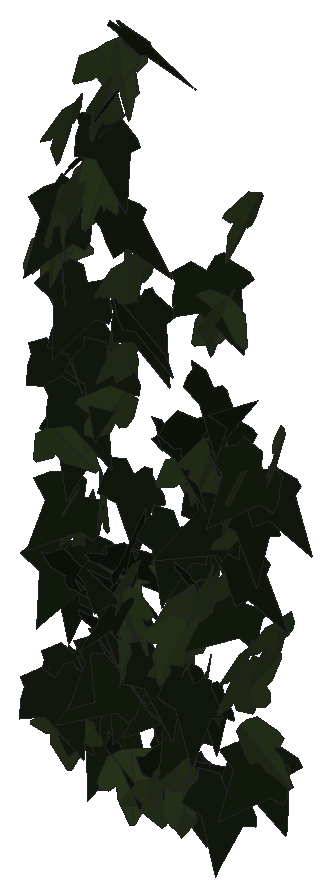
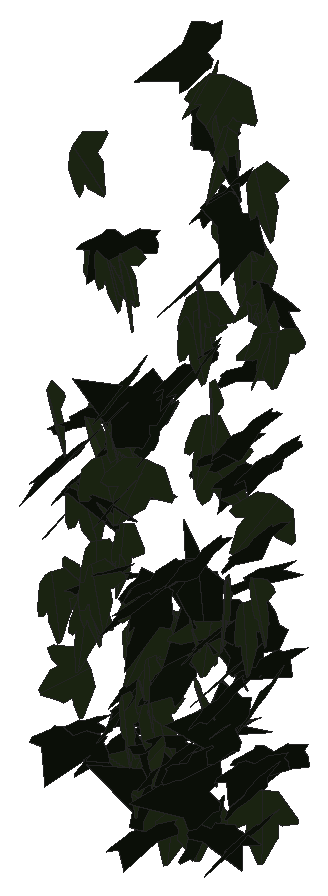
# SketchUp Ruby script. Lengths in inches.
U = 1.inch
M = Sketchup.active_model
def pt(a) = Geom::Point3d.new(a.map { |v| v * U })
def face(e, loops, mat)
  f = e.add_face(loops[0].map { |a| pt(a) })
  loops[1..].each { |l| e.add_face(l.map { |a| pt(a) }).erase! }
  f.material = f.back_material = mat if mat
  f
end
# faces: each face lists its corners as indices into pts; further lists are holes
def faces(e, pts, list, mat = nil) = list.each { |f| face(e, (f[0].is_a?(Array) ? f : [f]).map { |l| l.map { |i| pts[i] } }, mat) }
# xy, xz, yz: faces in a plane at the given z, y or x. An outline is a flat list of corners, or four numbers for a rectangle; further outlines are holes
def ring(l) = l.size == 4 ? [[l[0], l[1]], [l[2], l[1]], [l[2], l[3]], [l[0], l[3]]] : l.each_slice(2).to_a
def flat(e, list, mat, &to3) = list.each { |f| face(e, (f[0].is_a?(Array) ? f : [f]).map { |l| ring(l).map { |u, v| to3.(u, v) } }, mat) }
def xy(e, z, list, mat = nil) = flat(e, list, mat) { |x, y| [x, y, z] }
def xz(e, y, list, mat = nil) = flat(e, list, mat) { |x, z| [x, y, z] }
def yz(e, x, list, mat = nil) = flat(e, list, mat) { |y, z| [x, y, z] }
def lines(e, pts, list) = list.each { |a, b| e.add_line(pt(pts[a]), pt(pts[b])) }
# prism: a flat outline (further loops are holes) pulled along v
def prism(e, loops, v, mat = nil)
  f = face(e, loops, mat); d = Geom::Vector3d.new(v.map { |x| x * U })
  f.pushpull(f.normal.samedirection?(d) ? d.length : -d.length)
end
def box(e, o, s, mat = nil) = prism(e, [[o, [o[0] + s[0], o[1], o[2]], [o[0] + s[0], o[1] + s[1], o[2]], [o[0], o[1] + s[1], o[2]]]], [0, 0, s[2]], mat)
def at(x, y, z, deg = 0) = Geom::Transformation.translation(pt([x, y, z])) * Geom::Transformation.rotation(ORIGIN, Z_AXIS, deg.degrees)
def axes(o, x, y, z) = Geom::Transformation.new([*x, 0, *y, 0, *z, 0, *pt(o).to_a, 1])
def part(name) = M.definitions.add(name)
# library, detail: a bought-in or finely detailed component or shape, given as its bounding box
def library(name, o, s) = part(name).tap { |d| box(d.entities, o, s) }
def detail(e, o, s) = box(e.add_group.entities, o, s)
def put(e, d, t, mat = nil) = e.add_instance(d, t).tap { |i| i.material = mat if mat }
def group(e, t, mat = nil) = e.add_group.tap { |g| g.transformation = t; g.material = mat if mat }.entities
root = M.entities
M.materials.add("efeu1").color = [18, 25, 13]
M.materials.add("efeu2").color = [43, 57, 29]
c1 = part("ivyleaf_9")
p = [[1.54,2.16,1.25],[1.36,2.04,1.19],[-0.21,0.99,0.68],[-0.71,1.11,0.82],[-0.85,0.86,0.67],[-0.8,0.17,0.21],
  [-0.9,-0.01,0.1],[-0.67,-0.16,-0.02],[-0.08,-0.08,-0.05],[-0.03,-0.6,-0.4],[0.65,-0.88,-0.66],[0.83,-0.6,-0.49],
  [1.29,-0.42,-0.43],[1.8125,-0.07,-0.26],[1.21,0.44,0.15]]
faces(c1.entities,p,[[0,1,2,3,4,5,6,7,8,9,10,11,12,13,14]],"efeu1")
c2 = part("ivyleaf_10")
p = [[0,0.5,-0.03],[-0.0625,2.02,-0.43],[-0.19,2.01,-0.46],[-0.54,1.05,-0.29],[-0.52,0.625,-0.18],[-0.83,0.76,-0.28],
  [-1.16,0.64,-0.33],[-1.15,0.33,-0.24],[-0.77,-0.39,0.02],[-0.3,-0.51,0.16],[0.04,-0.48,0.23],[-0.02,2.01,-0.4375],
  [-0.06,2.01,-0.43],[0.04,-0.49,0.23],[0.67,-0.49,0.14],[1.38,0.36,-0.2],[1.375,0.51,-0.24],[0.81,0.65,-0.19],
  [0.62,0.59,-0.15],[0.6,1.09,-0.28],[0.5,1.23,-0.31]]
faces(c2.entities,p,[[0,1,2,3,4,5,6,7,8,9,10],[11,12,0,13,14,15,16,17,18,19,20]],"efeu2")
put(root,c1,axes([544.06,128.6,244.75],[-0.12791,-1.08437,0.12243],[0.01866,-0.12542,-1.09139],[1.0911,-0.12498,0.03302]))
put(root,c2,axes([544.82,128.41,258.1],[0.53643,-0.86378,0.36948],[0.17013,-0.32912,-1.01643],[0.92395,0.5621,-0.02735]))
put(root,c2,axes([544.29,128.17,265.42],[0.12998,-1.08128,0.03849],[-0.01205,-0.04022,-1.08894],[1.0819,0.12946,-0.01675]))
put(root,c2,axes([538.8,128.28,272.72],[0.35521,-1.05413,0.15556],[0.04081,-0.1504,-1.11233],[1.06476,0.35743,-0.00926]))
put(root,c2,axes([544.45,127.96,265.44],[0.92658,0.1574,-0.59669],[-0.61706,0.22347,-0.89926],[-0.00737,1.07919,0.27324]))
put(root,c2,axes([537.04,128.21,271],[0.14663,-1.11354,0.04185],[-0.00086,-0.04233,-1.12314],[1.11433,0.14649,-0.00637]))
put(root,c1,axes([536.51,128.12,247.02],[-0.11805,-0.83839,-0.60739],[0.19331,0.58272,-0.84192],[1.01708,-0.20806,0.08952]))
put(root,c1,axes([545.35,127.96,255.125],[0.64183,-0.75905,-0.41264],[-0.14061,0.41541,-0.98287],[0.85244,0.64004,0.14856]))
put(root,c1,axes([541.71,128.42,258.97],[0.6054,-0.84979,0.25487],[0.1449,-0.2097,-1.04338],[0.87527,0.62248,-0.00356]))
put(root,c2,axes([539.64,128.09,274.31],[-0.22158,1.08904,-0.20861],[0.06383,-0.19986,-1.11113],[-1.107,-0.22951,-0.02231]))
put(root,c1,axes([544.29,128.87,256.23],[-0.03542,-0.21643,-1.12372],[-0.13723,-1.11534,0.21915],[-1.13612,0.14147,0.00856]))
put(root,c1,axes([537.03,128.94,254.53],[-0.6452,-0.70565,0.47163],[-0.12229,-0.50895,-0.9288],[0.83989,-0.61618,0.22706]))
put(root,c1,axes([539.86,128.01,275.51],[0.97722,-0.56405,0.10988],[0.2353,0.195,-1.0917],[0.52427,0.96385,0.28516]))
put(root,c2,axes([543.68,127.95,253.52],[0.14871,-0.96486,-0.42015],[0.06481,0.43191,-0.96894],[1.05037,0.10995,0.11927]))
put(root,c2,axes([545.07,128.375,250.875],[0.25077,-1.00004,0.05704],[-0.00677,-0.06049,-1.03078],[1.00164,0.24996,-0.02125]))
put(root,c1,axes([537.21,128.92,263.54],[-0.42973,-0.96127,0.22537],[-0.02458,-0.2353,-1.05049],[0.98703,-0.42438,0.07196]))
put(root,c1,axes([539.66,128.32,251.56],[-0.89026,0.53258,-0.22377],[0.18218,-0.13129,-1.03724],[-0.54821,-0.90852,0.01871]))
put(root,c1,axes([538.99,128.98,247.5],[-0.84102,-0.46078,0.40771],[-0.17789,-0.47892,-0.90821],[0.58898,-0.8026,0.30786]))
put(root,c1,axes([543.51,128.28,266.49],[-0.03615,-0.87646,-0.66877],[0.25671,0.64404,-0.85793],[1.07216,-0.18375,0.18287]))
put(root,c1,axes([545.23,129.06,258.51],[-0.64176,-0.75796,0.41022],[-0.08164,-0.4557,-0.9697],[0.85797,-0.61031,0.21457]))
put(root,c1,axes([539.46,128.04,272.91],[-0.51577,0.9728,-0.16272],[0.10279,-0.12961,-1.10066],[-0.98094,-0.52507,-0.02978]))
put(root,c2,axes([538.88,128,274.15],[-0.73793,-0.66183,-0.54507],[0.41885,0.34924,-0.99109],[0.74813,-0.84834,0.01723]))
put(root,c1,axes([536.86,128.68,266.79],[-1.07208,-0.20445,-0.16315],[0.1581,0.04185,-1.09134],[0.20838,-1.08361,-0.01137]))
put(root,c2,axes([543.23,128.68,258.82],[-0.02355,-1.01285,0.35435],[0.08033,-0.3551,-1.00967],[1.07003,0.00436,0.08359]))
put(root,c2,axes([545.03,128.82,269.66],[0.17532,-0.94598,0.53413],[0.11746,-0.52136,-0.96192],[1.07998,0.21027,0.01791]))
put(root,c2,axes([539.61,128.36,251.43],[-0.91353,0.30764,-0.44243],[0.37507,-0.26225,-0.9568],[-0.38693,-0.98056,0.11709]))
put(root,c1,axes([536.84,128.4375,251.42],[0.37425,-0.36626,0.9382],[0.87748,-0.37272,-0.49553],[0.49437,0.93881,0.1693]))
put(root,c1,axes([542.35,128.88,248.48],[0.07802,-1.05092,0.15369],[-0.01944,-0.15549,-1.05337],[1.06192,0.07437,-0.03057]))
put(root,c2,axes([541.93,128.78,250.74],[-0.50453,-0.91681,0.45278],[-0.10124,-0.45763,-1.03944],[1.0175,-0.50014,0.1211]))
put(root,c1,axes([540.83,128.73,249.28],[0.1115,-1.04762,-0.20298],[-0.01522,0.2025,-1.05352],[1.06699,0.11237,0.00618]))
put(root,c2,axes([541.98,128.06,245.47],[-0.26892,-0.79208,-0.61992],[0.23526,0.57436,-0.83592],[0.97793,-0.35598,0.03062]))
put(root,c2,axes([538.25,128.58,268.55],[1.04573,-0.33669,-0.15025],[-0.14189,0.04957,-1.09859],[0.3403,1.0553,0.00366]))
put(root,c2,axes([545.14,128.28,250.08],[-0.04539,-0.98582,-0.46393],[0.07189,0.46061,-0.9858],[1.08715,-0.07162,0.04582]))
put(root,c1,axes([542.24,129.12,247.4],[-0.58299,-0.82912,0.08509],[-0.06149,-0.06078,-1.01345],[0.8312,-0.58603,-0.01529]))
put(root,c1,axes([538.22,128.87,270.52],[0.25197,-1.06277,-0.14593],[0.01988,0.1545,-1.09087],[1.07256,0.2468,0.0545]))
put(root,c2,axes([536.5625,128.29,257.37],[-0.69278,-0.5214,-0.62357],[0.55381,0.29695,-0.86357],[0.59498,-0.88352,0.07775]))
put(root,c2,axes([546.23,127.8125,250.49],[0.05579,-0.03913,1.05907],[-0.51266,0.9272,0.06126],[-0.92755,-0.51482,0.02984]))
put(root,c2,axes([536.1875,128.86,265.73],[-0.04701,0.96333,-0.52592],[-0.0558,-0.52782,-0.96182],[-1.09612,-0.01445,0.07152]))
put(root,c2,axes([543.23,128.53,265.22],[0.72169,-0.76625,-0.26758],[-0.09649,0.27452,-1.04638],[0.80587,0.71907,0.11434]))
put(root,c2,axes([539.44,128.94,252.22],[0.39845,-0.93808,0.28861],[0.07607,-0.28103,-1.01847],[0.97852,0.40383,-0.03835]))
put(root,c1,axes([539.29,128.69,252.63],[0.14082,0.85675,0.68004],[-0.1459,-0.66481,0.86778],[1.08406,-0.20077,0.02845]))
put(root,c1,axes([542.47,128.19,258.97],[0.13358,-0.24109,1.08514],[1.06427,0.34325,-0.05475],[-0.3209,1.03805,0.27013]))
put(root,c2,axes([545.33,128.67,247.57],[-0.74262,0.26915,-0.83997],[0.79373,-0.27496,-0.78985],[-0.38468,-1.08694,-0.00819]))
put(root,c2,axes([536.62,128.75,267.01],[-0.04822,1.05706,-0.31387],[-0.01638,-0.31482,-1.05775],[-1.10256,-0.04155,0.02944]))
put(root,c1,axes([537.04,128.71,259.22],[0.18352,-0.95892,-0.49518],[0.06149,0.51076,-0.96631],[1.07747,0.13418,0.13949]))
put(root,c2,axes([543.76,128.79,258.57],[0.67462,-0.84668,-0.05431],[-0.02693,0.04798,-1.08254],[0.84799,0.6751,0.00883]))
put(root,c2,axes([538.46,129.17,258.93],[-0.34573,-0.81918,0.59777],[-0.12062,-0.59385,-0.88358],[1.0069,-0.35242,0.09941]))
put(root,c2,axes([537.18,128.9,267.6],[0.24193,-1.06671,0.1041],[0.0008,-0.10654,-1.09357],[1.07178,0.24086,-0.02268]))
put(root,c1,axes([538.19,129.53,247.67],[-0.48604,-0.67717,0.61335],[-0.09813,-0.65202,-0.79763],[0.90836,-0.43277,0.24201]))
put(root,c2,axes([535.9375,128.63,264.91],[0.51737,0.95064,0.01218],[-0.03017,0.03027,-1.08153],[-0.95024,0.51663,0.04097]))
put(root,c2,axes([536.66,128.68,244.99],[-1.00531,-0.36923,0.13491],[-0.12852,-0.0414,-1.07095],[0.3715,-1.01347,-0.0054]))
put(root,c1,axes([544.1,129.55,252.24],[-0.68661,-0.62041,0.49026],[-0.14547,-0.5391,-0.88595],[0.77724,-0.64897,0.26728]))
put(root,c1,axes([535.92,129.01,260.16],[0.19128,-1.03022,-0.24829],[0.03319,0.25801,-1.04495],[1.0592,0.17796,0.07758]))
put(root,c2,axes([538.57,128.29,272.24],[0.19419,-0.8184,-0.74528],[0.07842,0.76493,-0.81955],[1.10411,0.08961,0.18929]))
put(root,c1,axes([536.08,129.49,251.46],[-0.4576,-0.91949,0.2445],[-0.01192,-0.26575,-1.0217],[0.95137,-0.4456,0.1048]))
put(root,c2,axes([537.01,128.68,268.05],[0.10966,-1.05379,-0.32369],[0.00392,0.32566,-1.05887],[1.10238,0.10367,0.03597]))
put(root,c2,axes([539.41,128.67,265.17],[-0.2633,-1.01234,-0.29769],[0.04781,0.29506,-1.04567],[1.05412,-0.26625,-0.02693]))
put(root,c2,axes([536.07,129.09,264.79],[-0.37733,0.88358,-0.52346],[0.16378,-0.49876,-0.95996],[-1.01386,-0.40942,0.03974]))
put(root,c2,axes([541.76,129.02,244.42],[-0.03996,-0.01063,1.12316],[1.12312,-0.01462,0.03982],[0.01424,1.12377,0.01114]))
put(root,c1,axes([544.58,129.4,256.6],[0.17037,-1.04692,0.13291],[0.03102,-0.1296,-1.06065],[1.05486,0.1729,0.00972]))
put(root,c1,axes([538.22,128.78,252.0625],[0.55765,-0.73407,-0.51362],[-0.04334,0.58218,-0.8791],[0.89486,0.48564,0.2775]))
put(root,c2,axes([536.57,128.99,254.33],[0.37404,-0.97216,-0.19561],[-0.07895,0.1792,-1.04159],[0.9885,0.38217,-0.00917]))
put(root,c1,axes([538.09,129.29,248.18],[0.6626,-0.66477,0.49589],[0.3453,-0.35597,-0.93857],[0.75406,0.74714,-0.00595]))
put(root,c1,axes([538.8,128.79,267.16],[0.71377,-0.70247,-0.44415],[-0.0956,0.51218,-0.96371],[0.82559,0.66664,0.2724]))
put(root,c1,axes([542.625,129.67,260.72],[0.16788,-0.94714,0.47533],[0.13502,-0.45822,-0.96073],[1.05108,0.21014,0.0475]))
put(root,c2,axes([544.55,129.27,255.69],[-0.15114,-1.04622,0.19358],[-0.02311,-0.19225,-1.05707],[1.06373,-0.15283,0.00454]))
put(root,c2,axes([538.99,129.22,249.01],[0.80031,-0.67786,0.0243],[0.00941,-0.02648,-1.04871],[0.67823,0.80024,-0.01412]))
put(root,c2,axes([541.25,129.38,249.07],[-0.07177,-0.97612,0.28866],[0.17783,-0.29695,-0.95994],[1.00225,-0.01721,0.19099]))
put(root,c1,axes([542.59,129.46,256.36],[0.29162,-1.00529,0.02952],[0.00865,-0.02823,-1.04673],[1.00569,0.29174,0.00044]))
put(root,c1,axes([538.73,128.53,252.87],[0.94996,0.53749,0.09691],[0.08472,0.04706,-1.09147],[-0.53954,0.95373,-0.00076]))
put(root,c1,axes([545,129.88,245.72],[-0.60946,-0.73971,0.37944],[-0.05654,-0.43251,-0.93398],[0.82942,-0.57302,0.21515]))
put(root,c2,axes([540.48,129.03,243.61],[-0.5643,-0.83663,-0.16183],[0.09172,0.13334,-1.00915],[0.84719,-0.5717,0.00146]))
put(root,c2,axes([539.27,129.32,264.6],[-0.04705,-1.08106,0.03747],[0.00002,-0.0375,-1.08208],[1.0817,-0.04702,0.00165]))
put(root,c1,axes([537.7,129.79,260.1],[-0.22955,-1.03616,0.0831],[-0.01383,-0.08205,-1.06127],[1.0394,-0.22992,0.00423]))
put(root,c1,axes([536.65,129.64,261.27],[0.04489,-1.06825,-0.05661],[-0.00063,0.05664,-1.06919],[1.06975,0.04486,0.00174]))
put(root,c2,axes([541.5,129.44,248.7],[0.53285,-0.9002,0.0656],[0.01589,-0.06681,-1.04589],[0.90245,0.5327,-0.02032]))
put(root,c2,axes([539.17,129.22,243.96],[0.7983,0.76395,0.04593],[0.03381,0.03111,-1.10495],[-0.76459,0.79901,-0.0009]))
put(root,c2,axes([541.89,128.57,243.06],[0.00809,0.67421,-0.8208],[0.04102,0.82001,0.67397],[1.06141,-0.03683,-0.01979]))
put(root,c2,axes([539.05,129.21,265.97],[0.75108,-0.76225,-0.19976],[0.03088,0.30423,-1.04477],[0.78739,0.71518,0.23153]))
put(root,c2,axes([541.84,129.07,251.97],[-0.37454,-0.88638,-0.36893],[0.11948,0.3499,-0.96195],[0.95263,-0.39238,-0.0244]))
put(root,c1,axes([535.71,129.99,250.19],[0.15262,-0.87701,0.5315],[0.09413,-0.52311,-0.89019],[1.02117,0.17929,0.00262]))
put(root,c2,axes([538.6,129.24,251.96],[0.66926,0.82232,0.12267],[0.06942,0.10166,-1.0602],[-0.82852,0.67278,0.01026]))
put(root,c2,axes([543.35,129.55,257.21],[-0.5407,-0.8953,0.20591],[-0.0641,-0.20159,-1.04479],[0.91644,-0.54233,0.04842]))
put(root,c1,axes([538.36,129.97,243.54],[0.2027,-0.74441,0.64559],[0.31374,-0.57604,-0.76273],[0.93408,0.35503,0.11609]))
put(root,c1,axes([540.75,129.16,243.89],[0.28907,-0.0248,1.07842],[1.06619,-0.16304,-0.28954],[0.16387,1.10452,-0.01853]))
put(root,c1,axes([537.68,128.57,269.6],[0.10664,0.98839,0.50155],[-0.03995,0.50697,-0.99057],[-1.10765,0.07688,0.08402]))
put(root,c1,axes([538.9,129.5,263.16],[0.666,-0.84486,-0.05222],[0.04952,0.10522,-1.07077],[0.84502,0.6597,0.1039]))
put(root,c2,axes([541.875,129.26,257.49],[-0.81745,-0.59294,-0.38587],[0.37871,0.13129,-1.00401],[0.59754,-0.89436,0.10844]))
put(root,c1,axes([536.22,130.16,246.21],[-0.11524,-0.88068,0.49667],[-0.02976,-0.49672,-0.88767],[1.01064,-0.11505,0.0305]))
put(root,c1,axes([539.29,129.53,263.1],[0.27064,-0.97158,-0.37476],[-0.01459,0.38363,-1.00512],[1.04125,0.25791,0.08332]))
put(root,c1,axes([536.07,130.1,256.8],[-0.11475,-1.02273,0.2172],[-0.00723,-0.21772,-1.02901],[1.04551,-0.11375,0.01672]))
put(root,c2,axes([541.47,129.03,250.78],[-0.24489,-0.78091,-0.68305],[0.24588,0.63814,-0.81772],[1.00793,-0.34541,0.03352]))
put(root,c1,axes([536.18,129.625,247.27],[0.0014,-0.92302,-0.46485],[0.13844,0.46082,-0.91462],[1.02415,-0.06103,0.12427]))
put(root,c1,axes([540.57,130.18,253.87],[-0.2085,-1.01226,0.15527],[-0.0021,-0.15804,-1.03309],[1.0241,-0.20642,0.02949]))
put(root,c2,axes([545.62,129.74,259.4],[0.56,-0.9002,0.01051],[0.01467,-0.00324,-1.06011],[0.90014,0.56009,0.01075]))
put(root,c2,axes([543.71,129.49,253.46],[-0.01225,-1.03038,-0.27187],[0.04624,0.27112,-1.02961],[1.06464,-0.02363,0.04159]))
put(root,c1,axes([543.55,130.12,256.23],[-0.84968,-0.49482,-0.3867],[0.44189,-0.00879,-0.95968],[0.44623,-0.93349,0.21402]))
put(root,c1,axes([538.56,130.12,255.41],[0.04517,-1.04483,0.03083],[0.00219,-0.03076,-1.04581],[1.04528,0.04521,0.00086]))
put(root,c1,axes([543.36,129.55,259.16],[0.62373,-0.76712,-0.4187],[-0.08076,0.4616,-0.96604],[0.87021,0.59268,0.21046]))
put(root,c1,axes([540.58,129.65,244.61],[-0.44615,0.5284,0.79464],[0.47066,-0.64124,0.69065],[0.83014,0.64754,0.03549]))
put(root,c1,axes([541.96,130.27,247.74],[0.23633,-0.9186,0.42702],[0.14628,-0.40295,-0.94777],[1.00239,0.27538,0.03764]))
put(root,c2,axes([545.54,129.75,251.63],[-0.05452,-1.04241,-0.06639],[0.00892,0.06602,-1.04382],[1.04449,-0.05497,0.00545]))
put(root,c2,axes([540.58,130.1,248.16],[0.03537,-0.98215,0.34089],[-0.00072,-0.34111,-0.98271],[1.03962,0.03318,-0.01228]))
put(root,c2,axes([541.01,129.6875,249.52],[0.28308,-0.97275,-0.25324],[-0.0155,0.25883,-1.01157],[1.00505,0.27797,0.05573]))
put(root,c2,axes([536.52,129.71,253.45],[0.17621,-1.02725,-0.2257],[0.00732,0.23004,-1.04128],[1.05173,0.17051,0.04506]))
put(root,c1,axes([541.04,129.43,252.73],[0.93346,0.12528,-0.48402],[-0.48578,-0.01528,-0.9408],[-0.11829,1.05137,0.04401]))
put(root,c2,axes([538.08,129.71,262.23],[0.49886,-0.8955,-0.3093],[-0.00064,0.34923,-1.01217],[0.94741,0.47177,0.16217]))
put(root,c1,axes([537.08,129.84,248.63],[0.76886,-0.37434,0.60056],[0.59504,-0.13804,-0.84783],[0.38305,0.9658,0.11159]))
put(root,c1,axes([540.37,130.6,247.15],[-0.77848,-0.58663,0.29971],[-0.08026,-0.37605,-0.94453],[0.65385,-0.74461,0.24089]))
put(root,c2,axes([543.41,130.03,252.82],[-0.04875,-1.04773,0.01676],[0.01491,-0.01747,-1.04875],[1.04776,-0.0485,0.0157]))
put(root,c1,axes([539.17,129.88,250.6],[0.94961,-0.4543,0.00246],[0.00219,-0.00113,-1.05268],[0.4543,0.94961,-0.00007]))
put(root,c2,axes([538.3125,129.82,260.82],[-0.09608,-0.99559,-0.36674],[0.13051,0.35436,-0.99615],[1.05293,-0.13477,0.09001]))
put(root,c1,axes([536.01,129.8125,244.75],[0.57356,-0.6952,-0.49424],[-0.07884,0.54983,-0.86488],[0.84933,0.52051,0.25349]))
put(root,c1,axes([537.45,130.47,244.44],[-0.7895,-0.5602,-0.24577],[0.22628,0.10537,-0.96708],[0.56836,-0.82013,0.04363]))
put(root,c1,axes([544.46,130.08,245.73],[-0.30217,-0.67484,-0.7262],[0.35284,0.63626,-0.73808],[0.92644,-0.46244,0.04424]))
put(root,c1,axes([544.9375,129.98,257.4],[0.47304,-0.82541,-0.45997],[-0.05449,0.4897,-0.93481],[0.94335,0.44219,0.17665]))
put(root,c1,axes([536.5,129.95,251.74],[0.63906,-0.7473,-0.39486],[-0.04179,0.46648,-0.95048],[0.84417,0.58882,0.25186]))
put(root,c1,axes([540.91,129.97,252.95],[0.46061,-0.80089,-0.4997],[0.06835,0.58285,-0.87115],[0.94151,0.3495,0.30771]))
put(root,c1,axes([538.39,130.7,247.08],[-0.44076,-0.92166,0.0783],[-0.02681,-0.07397,-1.0216],[0.92459,-0.44151,0.0077]))
put(root,c2,axes([537.16,129.99,254.41],[0.59897,-0.82304,-0.28597],[0.09855,0.40879,-0.97012],[0.86572,0.52291,0.30829]))
put(root,c1,axes([537.11,130.6,250.15],[0.12984,-1.01833,0.01596],[0.00003,-0.01609,-1.02657],[1.01846,0.12983,-0.002]))
put(root,c2,axes([541.68,130.35,248.02],[0.34243,-0.94102,-0.25436],[-0.04066,0.25558,-1.00025],[0.97395,0.34152,0.04767]))
put(root,c1,axes([539.23,130.96,246.84],[0.0192,-1.01634,0.02452],[0.00721,-0.02439,-1.0165],[1.01662,0.01937,0.00675]))
put(root,c1,axes([537.95,130.28,245.85],[0.87272,-0.11699,0.53583],[0.5442,0.05956,-0.87335],[0.06816,1.02236,0.1122]))
put(root,c2,axes([539.61,130.98,247.45],[-0.43935,0.58781,-0.70434],[0.41608,-0.56833,-0.73384],[-0.81761,-0.60508,0.00503]))
put(root,c1,axes([540.33,130.89,243.49],[0.00376,-0.93278,-0.39109],[0.13347,0.38813,-0.92444],[1.0026,-0.04817,0.12453]))
